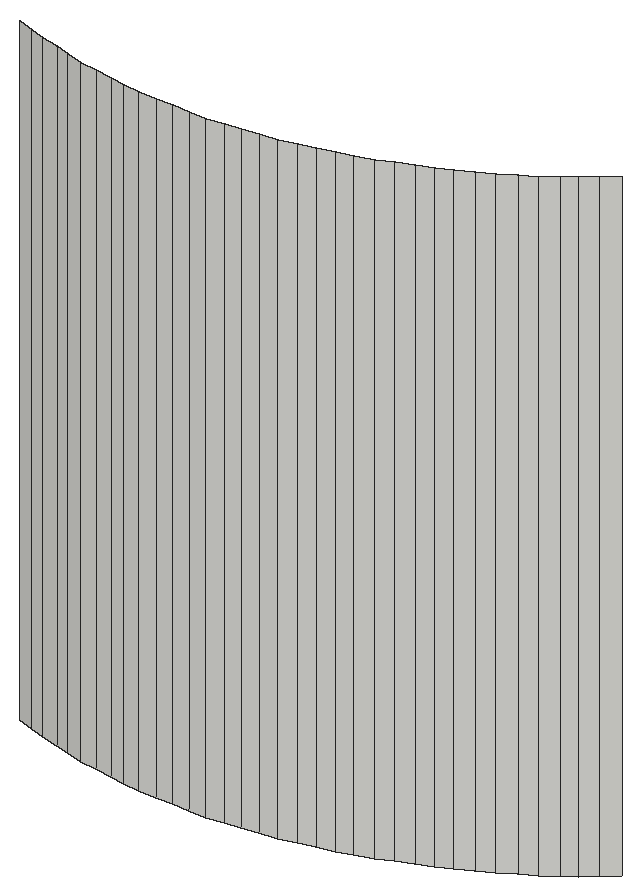
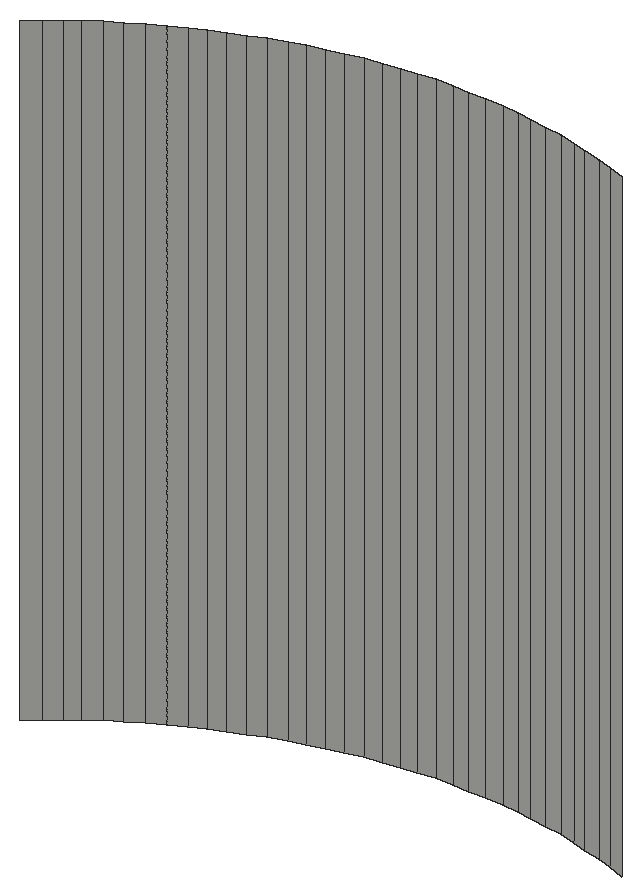
# SketchUp Ruby script. Lengths in inches.
U = 1.inch
M = Sketchup.active_model
def pt(a) = Geom::Point3d.new(a.map { |v| v * U })
def face(e, loops, mat)
  f = e.add_face(loops[0].map { |a| pt(a) })
  loops[1..].each { |l| e.add_face(l.map { |a| pt(a) }).erase! }
  f.material = f.back_material = mat if mat
  f
end
# faces: each face lists its corners as indices into pts; further lists are holes
def faces(e, pts, list, mat = nil) = list.each { |f| face(e, (f[0].is_a?(Array) ? f : [f]).map { |l| l.map { |i| pts[i] } }, mat) }
# xy, xz, yz: faces in a plane at the given z, y or x. An outline is a flat list of corners, or four numbers for a rectangle; further outlines are holes
def ring(l) = l.size == 4 ? [[l[0], l[1]], [l[2], l[1]], [l[2], l[3]], [l[0], l[3]]] : l.each_slice(2).to_a
def flat(e, list, mat, &to3) = list.each { |f| face(e, (f[0].is_a?(Array) ? f : [f]).map { |l| ring(l).map { |u, v| to3.(u, v) } }, mat) }
def xy(e, z, list, mat = nil) = flat(e, list, mat) { |x, y| [x, y, z] }
def xz(e, y, list, mat = nil) = flat(e, list, mat) { |x, z| [x, y, z] }
def yz(e, x, list, mat = nil) = flat(e, list, mat) { |y, z| [x, y, z] }
def lines(e, pts, list) = list.each { |a, b| e.add_line(pt(pts[a]), pt(pts[b])) }
# prism: a flat outline (further loops are holes) pulled along v
def prism(e, loops, v, mat = nil)
  f = face(e, loops, mat); d = Geom::Vector3d.new(v.map { |x| x * U })
  f.pushpull(f.normal.samedirection?(d) ? d.length : -d.length)
end
def box(e, o, s, mat = nil) = prism(e, [[o, [o[0] + s[0], o[1], o[2]], [o[0] + s[0], o[1] + s[1], o[2]], [o[0], o[1] + s[1], o[2]]]], [0, 0, s[2]], mat)
def at(x, y, z, deg = 0) = Geom::Transformation.translation(pt([x, y, z])) * Geom::Transformation.rotation(ORIGIN, Z_AXIS, deg.degrees)
def axes(o, x, y, z) = Geom::Transformation.new([*x, 0, *y, 0, *z, 0, *pt(o).to_a, 1])
def part(name) = M.definitions.add(name)
# library, detail: a bought-in or finely detailed component or shape, given as its bounding box
def library(name, o, s) = part(name).tap { |d| box(d.entities, o, s) }
def detail(e, o, s) = box(e.add_group.entities, o, s)
def put(e, d, t, mat = nil) = e.add_instance(d, t).tap { |i| i.material = mat if mat }
def group(e, t, mat = nil) = e.add_group.tap { |g| g.transformation = t; g.material = mat if mat }.entities
root = M.entities
xz(root,188.5,[[86.84,242,86.92,245],[86.92,242,87,245],[87,242,87.08,245],[87.08,242,87.16,245]])
p = [[86.53,188.54,242],[86.45,188.56,242],[86.45,188.56,245],[86.53,188.54,245],[86.61,188.53,242],[86.61,188.53,245],
  [86.6875,188.52,242],[86.6875,188.52,245],[86.76,188.51,242],[86.76,188.51,245],[86.84,188.5,242],[86.84,188.5,245],
  [87.24,188.51,242],[87.16,188.5,242],[87.16,188.5,245],[87.24,188.51,245],[87.3125,188.52,242],[87.3125,188.52,245],
  [87.39,188.53,242],[87.39,188.53,245],[87.47,188.54,242],[87.47,188.54,245],[87.55,188.56,242],[87.55,188.56,245],
  [86.23,188.62,242],[86.15,188.65,242],[86.15,188.65,245],[86.23,188.62,245],[86.3,188.6,242],[86.3,188.6,245],
  [86.38,188.58,242],[86.38,188.58,245],[87.62,188.58,242],[87.62,188.58,245],[87.7,188.6,242],[87.7,188.6,245],
  [87.77,188.62,242],[87.77,188.62,245],[87.85,188.65,242],[87.85,188.65,245],[87.92,188.68,242],[87.92,188.68,245],
  [87.99,188.71,242],[87.99,188.71,245],[88.0625,188.74,242],[88.0625,188.74,245],[88.13,188.77,242],[88.13,188.77,245],
  [88.2,188.81,242],[88.2,188.81,245],[88.27,188.85,242],[88.27,188.85,245],[88.34,188.89,242],[88.34,188.89,245],
  [88.41,188.93,242],[88.41,188.93,245],[88.47,188.98,242],[88.47,188.98,245],[88.53,189.02,242],[88.53,189.02,245],
  [88.59,189.07,242],[88.59,189.07,245],[88.65,189.125,242],[88.65,189.125,245]]
faces(root,p,[[0,1,2,3],[4,0,3,5],[6,4,5,7],[8,6,7,9],[10,8,9,11],[12,13,14,15],[16,12,15,17],[18,16,17,19],
  [20,18,19,21],[22,20,21,23],[24,25,26,27],[28,24,27,29],[30,28,29,31],[1,30,31,2],[32,22,23,33],[34,32,33,35],
  [36,34,35,37],[38,36,37,39],[40,38,39,41],[42,40,41,43],[44,42,43,45],[46,44,45,47],[48,46,47,49],[50,48,49,51],
  [52,50,51,53],[54,52,53,55],[56,54,55,57],[58,56,57,59],[60,58,59,61],[62,60,61,63]])
